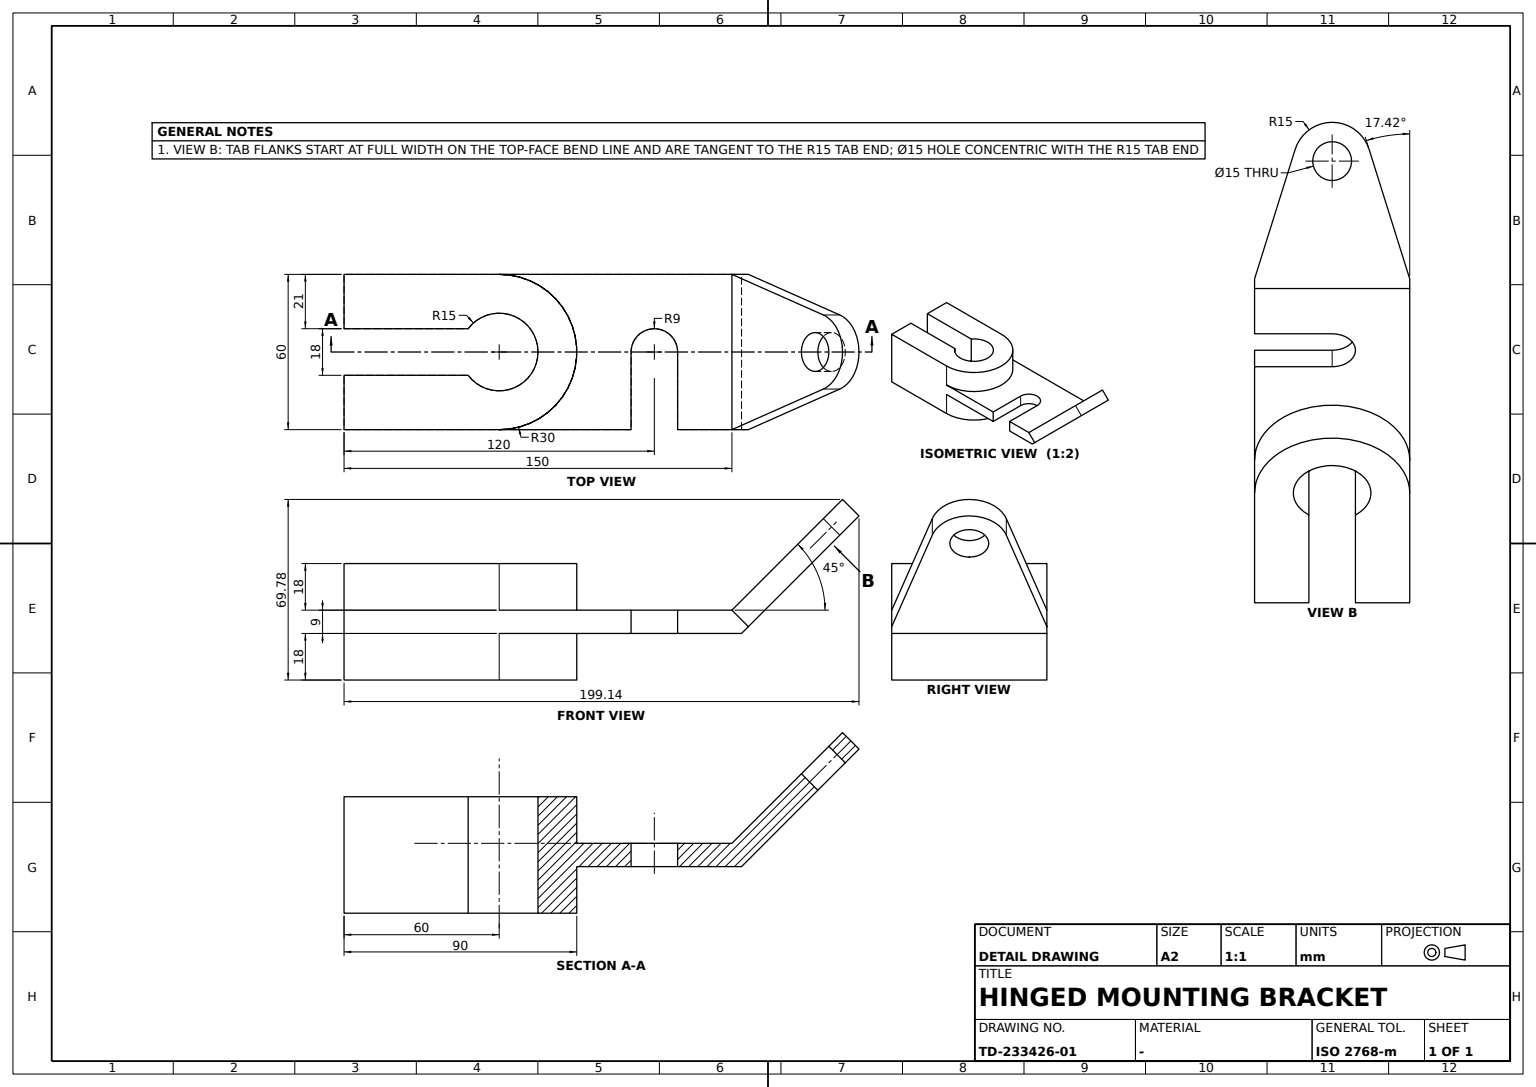
ISO-10303-21;
HEADER;
FILE_DESCRIPTION((''),'2;1');
FILE_NAME('','',(''),(''),'','','');
FILE_SCHEMA(('AUTOMOTIVE_DESIGN'));
ENDSEC;
DATA;
#1=APPLICATION_CONTEXT('');
#2=PRODUCT_CONTEXT('',#1,'mechanical');
#3=PRODUCT('','','',(#2));
#4=PRODUCT_DEFINITION_FORMATION('','',#3);
#5=PRODUCT_DEFINITION_CONTEXT('',#1,'design');
#6=PRODUCT_DEFINITION('','',#4,#5);
#7=PRODUCT_DEFINITION_SHAPE('','',#6);
#8=(LENGTH_UNIT()NAMED_UNIT(*)SI_UNIT(.MILLI.,.METRE.));
#9=(NAMED_UNIT(*)PLANE_ANGLE_UNIT()SI_UNIT($,.RADIAN.));
#10=(NAMED_UNIT(*)SI_UNIT($,.STERADIAN.)SOLID_ANGLE_UNIT());
#11=UNCERTAINTY_MEASURE_WITH_UNIT(LENGTH_MEASURE(0.005),#8,'distance_accuracy_value','');
#12=(GEOMETRIC_REPRESENTATION_CONTEXT(3)GLOBAL_UNCERTAINTY_ASSIGNED_CONTEXT((#11))GLOBAL_UNIT_ASSIGNED_CONTEXT((#8,#9,#10))REPRESENTATION_CONTEXT('',''));
#13=CARTESIAN_POINT('',(132.77996,0.,47.27996));
#14=VERTEX_POINT('',#13);
#15=CARTESIAN_POINT('',(125.349193,14.311818,39.849193));
#16=VERTEX_POINT('',#15);
#17=CARTESIAN_POINT('',(122.173359,0.,36.673359));
#18=DIRECTION('',(-0.707106781,0.,0.707106781));
#19=DIRECTION('',(0.707106781,0.,0.707106781));
#20=AXIS2_PLACEMENT_3D('',#17,#18,#19);
#21=CIRCLE('',#20,15.);
#22=EDGE_CURVE('',#14,#16,#21,.T.);
#23=ORIENTED_EDGE('',*,*,#22,.T.);
#24=CARTESIAN_POINT('',(90.,30.,4.5));
#25=VERTEX_POINT('',#24);
#26=DIRECTION('',(0.674665588,-0.299420588,0.674665588));
#27=VECTOR('',#26,1000.);
#28=LINE('',#24,#27);
#29=EDGE_CURVE('',#25,#16,#28,.T.);
#30=ORIENTED_EDGE('',*,*,#29,.F.);
#31=CARTESIAN_POINT('',(90.,-30.,4.5));
#32=VERTEX_POINT('',#31);
#33=DIRECTION('',(0.,1.,0.));
#34=VECTOR('',#33,1000.);
#35=LINE('',#31,#34);
#36=EDGE_CURVE('',#32,#25,#35,.T.);
#37=ORIENTED_EDGE('',*,*,#36,.F.);
#38=CARTESIAN_POINT('',(125.349193,-14.311818,39.849193));
#39=VERTEX_POINT('',#38);
#40=DIRECTION('',(-0.674665588,-0.299420588,-0.674665588));
#41=VECTOR('',#40,1000.);
#42=LINE('',#38,#41);
#43=EDGE_CURVE('',#39,#32,#42,.T.);
#44=ORIENTED_EDGE('',*,*,#43,.F.);
#45=EDGE_CURVE('',#39,#14,#21,.T.);
#46=ORIENTED_EDGE('',*,*,#45,.T.);
#47=EDGE_LOOP('',(#23,#30,#37,#44,#46));
#48=FACE_BOUND('',#47,.T.);
#49=CARTESIAN_POINT('',(127.476659,0.,41.976659));
#50=VERTEX_POINT('',#49);
#51=CARTESIAN_POINT('',(116.870058,0.,31.370058));
#52=VERTEX_POINT('',#51);
#53=AXIS2_PLACEMENT_3D('',#17,#18,#26);
#54=CIRCLE('',#53,7.5);
#55=EDGE_CURVE('',#50,#52,#54,.T.);
#56=ORIENTED_EDGE('',*,*,#55,.F.);
#57=EDGE_CURVE('',#52,#50,#54,.T.);
#58=ORIENTED_EDGE('',*,*,#57,.F.);
#59=EDGE_LOOP('',(#56,#58));
#60=FACE_BOUND('',#59,.T.);
#61=CARTESIAN_POINT('',(116.870058,-30.,31.370058));
#62=DIRECTION('',(0.707106781,0.,-0.707106781));
#63=DIRECTION('',(-0.707106781,0.,-0.707106781));
#64=AXIS2_PLACEMENT_3D('',#61,#62,#63);
#65=PLANE('',#64);
#66=ADVANCED_FACE('',(#48,#60),#65,.F.);
#67=ORIENTED_EDGE('',*,*,#55,.T.);
#68=CARTESIAN_POINT('',(123.234019,0.,25.006097));
#69=VERTEX_POINT('',#68);
#70=VECTOR('',#18,1000.);
#71=LINE('',#68,#70);
#72=EDGE_CURVE('',#69,#52,#71,.T.);
#73=ORIENTED_EDGE('',*,*,#72,.F.);
#74=CARTESIAN_POINT('',(133.84062,0.,35.612698));
#75=VERTEX_POINT('',#74);
#76=CARTESIAN_POINT('',(128.53732,0.,30.309398));
#77=AXIS2_PLACEMENT_3D('',#76,#18,#26);
#78=CIRCLE('',#77,7.5);
#79=EDGE_CURVE('',#75,#69,#78,.T.);
#80=ORIENTED_EDGE('',*,*,#79,.F.);
#81=LINE('',#74,#70);
#82=EDGE_CURVE('',#50,#75,#81,.F.);
#83=ORIENTED_EDGE('',*,*,#82,.F.);
#84=EDGE_LOOP('',(#67,#73,#80,#83));
#85=FACE_BOUND('',#84,.T.);
#86=AXIS2_PLACEMENT_3D('',#76,#18,#19);
#87=CYLINDRICAL_SURFACE('',#86,7.5);
#88=ADVANCED_FACE('',(#85),#87,.F.);
#89=CARTESIAN_POINT('',(51.,-30.,-4.5));
#90=VERTEX_POINT('',#89);
#91=CARTESIAN_POINT('',(51.,-30.,4.5));
#92=VERTEX_POINT('',#91);
#93=CARTESIAN_POINT('',(51.,-30.,-55.5));
#94=DIRECTION('',(0.,0.,1.));
#95=VECTOR('',#94,1000.);
#96=LINE('',#93,#95);
#97=EDGE_CURVE('',#90,#92,#96,.T.);
#98=ORIENTED_EDGE('',*,*,#97,.T.);
#99=CARTESIAN_POINT('',(0.,-30.,4.5));
#100=VERTEX_POINT('',#99);
#101=DIRECTION('',(-1.,0.,0.));
#102=VECTOR('',#101,1000.);
#103=LINE('',#31,#102);
#104=EDGE_CURVE('',#92,#100,#103,.T.);
#105=ORIENTED_EDGE('',*,*,#104,.T.);
#106=CARTESIAN_POINT('',(0.,-30.,22.5));
#107=VERTEX_POINT('',#106);
#108=DIRECTION('',(0.,0.,-1.));
#109=VECTOR('',#108,1000.);
#110=LINE('',#106,#109);
#111=EDGE_CURVE('',#107,#100,#110,.T.);
#112=ORIENTED_EDGE('',*,*,#111,.F.);
#113=CARTESIAN_POINT('',(-60.,-30.,22.5));
#114=VERTEX_POINT('',#113);
#115=DIRECTION('',(1.,0.,0.));
#116=VECTOR('',#115,1000.);
#117=LINE('',#113,#116);
#118=EDGE_CURVE('',#114,#107,#117,.T.);
#119=ORIENTED_EDGE('',*,*,#118,.F.);
#120=CARTESIAN_POINT('',(-60.,-30.,-22.5));
#121=VERTEX_POINT('',#120);
#122=LINE('',#113,#109);
#123=EDGE_CURVE('',#114,#121,#122,.T.);
#124=ORIENTED_EDGE('',*,*,#123,.T.);
#125=CARTESIAN_POINT('',(0.,-30.,-22.5));
#126=VERTEX_POINT('',#125);
#127=LINE('',#120,#116);
#128=EDGE_CURVE('',#121,#126,#127,.T.);
#129=ORIENTED_EDGE('',*,*,#128,.T.);
#130=CARTESIAN_POINT('',(0.,-30.,-4.5));
#131=VERTEX_POINT('',#130);
#132=EDGE_CURVE('',#131,#126,#110,.T.);
#133=ORIENTED_EDGE('',*,*,#132,.F.);
#134=LINE('',#130,#116);
#135=EDGE_CURVE('',#131,#90,#134,.T.);
#136=ORIENTED_EDGE('',*,*,#135,.T.);
#137=EDGE_LOOP('',(#98,#105,#112,#119,#124,#129,#133,#136));
#138=FACE_BOUND('',#137,.T.);
#139=AXIS2_PLACEMENT_3D('',#113,#33,#94);
#140=PLANE('',#139);
#141=ADVANCED_FACE('',(#138),#140,.F.);
#142=CARTESIAN_POINT('',(69.,0.,4.5));
#143=VERTEX_POINT('',#142);
#144=CARTESIAN_POINT('',(51.,0.,4.5));
#145=VERTEX_POINT('',#144);
#146=CARTESIAN_POINT('',(60.,0.,4.5));
#147=AXIS2_PLACEMENT_3D('',#146,#94,#115);
#148=CIRCLE('',#147,9.);
#149=EDGE_CURVE('',#143,#145,#148,.T.);
#150=ORIENTED_EDGE('',*,*,#149,.F.);
#151=CARTESIAN_POINT('',(69.,-30.,4.5));
#152=VERTEX_POINT('',#151);
#153=LINE('',#151,#34);
#154=EDGE_CURVE('',#152,#143,#153,.T.);
#155=ORIENTED_EDGE('',*,*,#154,.F.);
#156=EDGE_CURVE('',#32,#152,#103,.T.);
#157=ORIENTED_EDGE('',*,*,#156,.F.);
#158=ORIENTED_EDGE('',*,*,#36,.T.);
#159=CARTESIAN_POINT('',(0.,30.,4.5));
#160=VERTEX_POINT('',#159);
#161=LINE('',#24,#102);
#162=EDGE_CURVE('',#25,#160,#161,.T.);
#163=ORIENTED_EDGE('',*,*,#162,.T.);
#164=CARTESIAN_POINT('',(0.,0.,4.5));
#165=AXIS2_PLACEMENT_3D('',#164,#108,#101);
#166=CIRCLE('',#165,30.);
#167=EDGE_CURVE('',#160,#100,#166,.T.);
#168=ORIENTED_EDGE('',*,*,#167,.T.);
#169=ORIENTED_EDGE('',*,*,#104,.F.);
#170=DIRECTION('',(0.,-1.,0.));
#171=VECTOR('',#170,1000.);
#172=LINE('',#144,#171);
#173=EDGE_CURVE('',#145,#92,#172,.T.);
#174=ORIENTED_EDGE('',*,*,#173,.F.);
#175=EDGE_LOOP('',(#150,#155,#157,#158,#163,#168,#169,#174));
#176=FACE_BOUND('',#175,.T.);
#177=AXIS2_PLACEMENT_3D('',#31,#108,#101);
#178=PLANE('',#177);
#179=ADVANCED_FACE('',(#176),#178,.F.);
#180=ORIENTED_EDGE('',*,*,#79,.T.);
#181=EDGE_CURVE('',#69,#75,#78,.T.);
#182=ORIENTED_EDGE('',*,*,#181,.T.);
#183=EDGE_LOOP('',(#180,#182));
#184=FACE_BOUND('',#183,.T.);
#185=CARTESIAN_POINT('',(93.727922,-30.,-4.5));
#186=VERTEX_POINT('',#185);
#187=CARTESIAN_POINT('',(96.363961,-30.,-1.863961));
#188=VERTEX_POINT('',#187);
#189=VECTOR('',#19,1000.);
#190=LINE('',#185,#189);
#191=EDGE_CURVE('',#186,#188,#190,.T.);
#192=ORIENTED_EDGE('',*,*,#191,.F.);
#193=CARTESIAN_POINT('',(93.727922,30.,-4.5));
#194=VERTEX_POINT('',#193);
#195=LINE('',#185,#34);
#196=EDGE_CURVE('',#186,#194,#195,.T.);
#197=ORIENTED_EDGE('',*,*,#196,.T.);
#198=CARTESIAN_POINT('',(96.363961,30.,-1.863961));
#199=VERTEX_POINT('',#198);
#200=LINE('',#193,#189);
#201=EDGE_CURVE('',#194,#199,#200,.T.);
#202=ORIENTED_EDGE('',*,*,#201,.T.);
#203=CARTESIAN_POINT('',(131.713154,14.311818,33.485232));
#204=VERTEX_POINT('',#203);
#205=LINE('',#198,#27);
#206=EDGE_CURVE('',#199,#204,#205,.T.);
#207=ORIENTED_EDGE('',*,*,#206,.T.);
#208=CARTESIAN_POINT('',(139.143921,0.,40.915999));
#209=VERTEX_POINT('',#208);
#210=CIRCLE('',#86,15.);
#211=EDGE_CURVE('',#209,#204,#210,.T.);
#212=ORIENTED_EDGE('',*,*,#211,.F.);
#213=CARTESIAN_POINT('',(131.713154,-14.311818,33.485232));
#214=VERTEX_POINT('',#213);
#215=EDGE_CURVE('',#214,#209,#210,.T.);
#216=ORIENTED_EDGE('',*,*,#215,.F.);
#217=LINE('',#213,#41);
#218=EDGE_CURVE('',#214,#188,#217,.T.);
#219=ORIENTED_EDGE('',*,*,#218,.T.);
#220=EDGE_LOOP('',(#192,#197,#202,#207,#212,#216,#219));
#221=FACE_BOUND('',#220,.T.);
#222=AXIS2_PLACEMENT_3D('',#185,#18,#19);
#223=PLANE('',#222);
#224=ADVANCED_FACE('',(#184,#221),#223,.F.);
#225=CARTESIAN_POINT('',(-12.,9.,-22.5));
#226=VERTEX_POINT('',#225);
#227=CARTESIAN_POINT('',(-60.,9.,-22.5));
#228=VERTEX_POINT('',#227);
#229=CARTESIAN_POINT('',(8.,9.,-22.5));
#230=LINE('',#229,#102);
#231=EDGE_CURVE('',#226,#228,#230,.T.);
#232=ORIENTED_EDGE('',*,*,#231,.T.);
#233=CARTESIAN_POINT('',(-60.,30.,-22.5));
#234=VERTEX_POINT('',#233);
#235=LINE('',#233,#171);
#236=EDGE_CURVE('',#234,#228,#235,.T.);
#237=ORIENTED_EDGE('',*,*,#236,.F.);
#238=CARTESIAN_POINT('',(0.,30.,-22.5));
#239=VERTEX_POINT('',#238);
#240=LINE('',#238,#102);
#241=EDGE_CURVE('',#239,#234,#240,.T.);
#242=ORIENTED_EDGE('',*,*,#241,.F.);
#243=CARTESIAN_POINT('',(0.,0.,-22.5));
#244=AXIS2_PLACEMENT_3D('',#243,#94,#115);
#245=CIRCLE('',#244,30.);
#246=EDGE_CURVE('',#126,#239,#245,.T.);
#247=ORIENTED_EDGE('',*,*,#246,.F.);
#248=ORIENTED_EDGE('',*,*,#128,.F.);
#249=CARTESIAN_POINT('',(-60.,-9.,-22.5));
#250=VERTEX_POINT('',#249);
#251=EDGE_CURVE('',#250,#121,#235,.T.);
#252=ORIENTED_EDGE('',*,*,#251,.F.);
#253=CARTESIAN_POINT('',(-12.,-9.,-22.5));
#254=VERTEX_POINT('',#253);
#255=LINE('',#249,#116);
#256=EDGE_CURVE('',#250,#254,#255,.T.);
#257=ORIENTED_EDGE('',*,*,#256,.T.);
#258=CARTESIAN_POINT('',(15.,0.,-22.5));
#259=VERTEX_POINT('',#258);
#260=AXIS2_PLACEMENT_3D('',#243,#94,#33);
#261=CIRCLE('',#260,15.);
#262=EDGE_CURVE('',#254,#259,#261,.T.);
#263=ORIENTED_EDGE('',*,*,#262,.T.);
#264=EDGE_CURVE('',#259,#226,#261,.T.);
#265=ORIENTED_EDGE('',*,*,#264,.T.);
#266=EDGE_LOOP('',(#232,#237,#242,#247,#248,#252,#257,#263,#265));
#267=FACE_BOUND('',#266,.T.);
#268=PLANE('',#244);
#269=ADVANCED_FACE('',(#267),#268,.F.);
#270=CARTESIAN_POINT('',(0.,30.,22.5));
#271=VERTEX_POINT('',#270);
#272=LINE('',#270,#109);
#273=EDGE_CURVE('',#271,#160,#272,.T.);
#274=ORIENTED_EDGE('',*,*,#273,.F.);
#275=CARTESIAN_POINT('',(0.,0.,22.5));
#276=AXIS2_PLACEMENT_3D('',#275,#94,#115);
#277=CIRCLE('',#276,30.);
#278=EDGE_CURVE('',#107,#271,#277,.T.);
#279=ORIENTED_EDGE('',*,*,#278,.F.);
#280=ORIENTED_EDGE('',*,*,#111,.T.);
#281=ORIENTED_EDGE('',*,*,#167,.F.);
#282=EDGE_LOOP('',(#274,#279,#280,#281));
#283=FACE_BOUND('',#282,.T.);
#284=AXIS2_PLACEMENT_3D('',#275,#108,#101);
#285=CYLINDRICAL_SURFACE('',#284,30.);
#286=ADVANCED_FACE('',(#283),#285,.T.);
#287=ORIENTED_EDGE('',*,*,#29,.T.);
#288=LINE('',#203,#70);
#289=EDGE_CURVE('',#204,#16,#288,.T.);
#290=ORIENTED_EDGE('',*,*,#289,.F.);
#291=ORIENTED_EDGE('',*,*,#206,.F.);
#292=LINE('',#198,#70);
#293=EDGE_CURVE('',#199,#25,#292,.T.);
#294=ORIENTED_EDGE('',*,*,#293,.T.);
#295=EDGE_LOOP('',(#287,#290,#291,#294));
#296=FACE_BOUND('',#295,.T.);
#297=DIRECTION('',(-0.211722328,-0.954121225,-0.211722328));
#298=DIRECTION('',(0.976253017,-0.216633438,0.));
#299=AXIS2_PLACEMENT_3D('',#198,#297,#298);
#300=PLANE('',#299);
#301=ADVANCED_FACE('',(#296),#300,.F.);
#302=CARTESIAN_POINT('',(0.,30.,-4.5));
#303=VERTEX_POINT('',#302);
#304=EDGE_CURVE('',#303,#239,#272,.T.);
#305=ORIENTED_EDGE('',*,*,#304,.T.);
#306=ORIENTED_EDGE('',*,*,#241,.T.);
#307=CARTESIAN_POINT('',(-60.,30.,22.5));
#308=VERTEX_POINT('',#307);
#309=LINE('',#307,#109);
#310=EDGE_CURVE('',#308,#234,#309,.T.);
#311=ORIENTED_EDGE('',*,*,#310,.F.);
#312=LINE('',#270,#102);
#313=EDGE_CURVE('',#271,#308,#312,.T.);
#314=ORIENTED_EDGE('',*,*,#313,.F.);
#315=ORIENTED_EDGE('',*,*,#273,.T.);
#316=ORIENTED_EDGE('',*,*,#162,.F.);
#317=ORIENTED_EDGE('',*,*,#293,.F.);
#318=ORIENTED_EDGE('',*,*,#201,.F.);
#319=LINE('',#302,#116);
#320=EDGE_CURVE('',#303,#194,#319,.T.);
#321=ORIENTED_EDGE('',*,*,#320,.F.);
#322=EDGE_LOOP('',(#305,#306,#311,#314,#315,#316,#317,#318,#321));
#323=FACE_BOUND('',#322,.T.);
#324=AXIS2_PLACEMENT_3D('',#270,#170,#108);
#325=PLANE('',#324);
#326=ADVANCED_FACE('',(#323),#325,.F.);
#327=ORIENTED_EDGE('',*,*,#231,.F.);
#328=CARTESIAN_POINT('',(-12.,9.,22.5));
#329=VERTEX_POINT('',#328);
#330=LINE('',#225,#109);
#331=EDGE_CURVE('',#329,#226,#330,.T.);
#332=ORIENTED_EDGE('',*,*,#331,.F.);
#333=CARTESIAN_POINT('',(-60.,9.,22.5));
#334=VERTEX_POINT('',#333);
#335=CARTESIAN_POINT('',(8.,9.,22.5));
#336=LINE('',#335,#102);
#337=EDGE_CURVE('',#329,#334,#336,.T.);
#338=ORIENTED_EDGE('',*,*,#337,.T.);
#339=LINE('',#227,#95);
#340=EDGE_CURVE('',#228,#334,#339,.T.);
#341=ORIENTED_EDGE('',*,*,#340,.F.);
#342=EDGE_LOOP('',(#327,#332,#338,#341));
#343=FACE_BOUND('',#342,.T.);
#344=AXIS2_PLACEMENT_3D('',#229,#33,#101);
#345=PLANE('',#344);
#346=ADVANCED_FACE('',(#343),#345,.F.);
#347=ORIENTED_EDGE('',*,*,#246,.T.);
#348=ORIENTED_EDGE('',*,*,#304,.F.);
#349=CARTESIAN_POINT('',(0.,0.,-4.5));
#350=AXIS2_PLACEMENT_3D('',#349,#94,#115);
#351=CIRCLE('',#350,30.);
#352=EDGE_CURVE('',#131,#303,#351,.T.);
#353=ORIENTED_EDGE('',*,*,#352,.F.);
#354=ORIENTED_EDGE('',*,*,#132,.T.);
#355=EDGE_LOOP('',(#347,#348,#353,#354));
#356=FACE_BOUND('',#355,.T.);
#357=ADVANCED_FACE('',(#356),#285,.T.);
#358=ORIENTED_EDGE('',*,*,#57,.T.);
#359=ORIENTED_EDGE('',*,*,#82,.T.);
#360=ORIENTED_EDGE('',*,*,#181,.F.);
#361=ORIENTED_EDGE('',*,*,#72,.T.);
#362=EDGE_LOOP('',(#358,#359,#360,#361));
#363=FACE_BOUND('',#362,.T.);
#364=ADVANCED_FACE('',(#363),#87,.F.);
#365=CARTESIAN_POINT('',(-12.,-9.,22.5));
#366=VERTEX_POINT('',#365);
#367=LINE('',#253,#95);
#368=EDGE_CURVE('',#254,#366,#367,.T.);
#369=ORIENTED_EDGE('',*,*,#368,.F.);
#370=ORIENTED_EDGE('',*,*,#256,.F.);
#371=CARTESIAN_POINT('',(-60.,-9.,22.5));
#372=VERTEX_POINT('',#371);
#373=LINE('',#249,#95);
#374=EDGE_CURVE('',#250,#372,#373,.T.);
#375=ORIENTED_EDGE('',*,*,#374,.T.);
#376=LINE('',#371,#116);
#377=EDGE_CURVE('',#372,#366,#376,.T.);
#378=ORIENTED_EDGE('',*,*,#377,.T.);
#379=EDGE_LOOP('',(#369,#370,#375,#378));
#380=FACE_BOUND('',#379,.T.);
#381=AXIS2_PLACEMENT_3D('',#249,#170,#115);
#382=PLANE('',#381);
#383=ADVANCED_FACE('',(#380),#382,.F.);
#384=CARTESIAN_POINT('',(51.,0.,-4.5));
#385=VERTEX_POINT('',#384);
#386=CARTESIAN_POINT('',(51.,0.,-55.5));
#387=LINE('',#386,#109);
#388=EDGE_CURVE('',#145,#385,#387,.T.);
#389=ORIENTED_EDGE('',*,*,#388,.F.);
#390=ORIENTED_EDGE('',*,*,#173,.T.);
#391=ORIENTED_EDGE('',*,*,#97,.F.);
#392=LINE('',#89,#171);
#393=EDGE_CURVE('',#385,#90,#392,.T.);
#394=ORIENTED_EDGE('',*,*,#393,.F.);
#395=EDGE_LOOP('',(#389,#390,#391,#394));
#396=FACE_BOUND('',#395,.T.);
#397=AXIS2_PLACEMENT_3D('',#386,#101,#170);
#398=PLANE('',#397);
#399=ADVANCED_FACE('',(#396),#398,.F.);
#400=ORIENTED_EDGE('',*,*,#236,.T.);
#401=ORIENTED_EDGE('',*,*,#340,.T.);
#402=LINE('',#307,#171);
#403=EDGE_CURVE('',#308,#334,#402,.T.);
#404=ORIENTED_EDGE('',*,*,#403,.F.);
#405=ORIENTED_EDGE('',*,*,#310,.T.);
#406=EDGE_LOOP('',(#400,#401,#404,#405));
#407=FACE_BOUND('',#406,.T.);
#408=AXIS2_PLACEMENT_3D('',#307,#115,#108);
#409=PLANE('',#408);
#410=ADVANCED_FACE('',(#407),#409,.F.);
#411=ORIENTED_EDGE('',*,*,#374,.F.);
#412=ORIENTED_EDGE('',*,*,#251,.T.);
#413=ORIENTED_EDGE('',*,*,#123,.F.);
#414=EDGE_CURVE('',#372,#114,#402,.T.);
#415=ORIENTED_EDGE('',*,*,#414,.F.);
#416=EDGE_LOOP('',(#411,#412,#413,#415));
#417=FACE_BOUND('',#416,.T.);
#418=ADVANCED_FACE('',(#417),#409,.F.);
#419=CARTESIAN_POINT('',(15.,0.,22.5));
#420=VERTEX_POINT('',#419);
#421=AXIS2_PLACEMENT_3D('',#275,#94,#33);
#422=CIRCLE('',#421,15.);
#423=EDGE_CURVE('',#366,#420,#422,.T.);
#424=ORIENTED_EDGE('',*,*,#423,.T.);
#425=LINE('',#258,#95);
#426=EDGE_CURVE('',#259,#420,#425,.T.);
#427=ORIENTED_EDGE('',*,*,#426,.F.);
#428=ORIENTED_EDGE('',*,*,#262,.F.);
#429=ORIENTED_EDGE('',*,*,#368,.T.);
#430=EDGE_LOOP('',(#424,#427,#428,#429));
#431=FACE_BOUND('',#430,.T.);
#432=CYLINDRICAL_SURFACE('',#244,15.);
#433=ADVANCED_FACE('',(#431),#432,.F.);
#434=ORIENTED_EDGE('',*,*,#22,.F.);
#435=LINE('',#208,#70);
#436=EDGE_CURVE('',#209,#14,#435,.T.);
#437=ORIENTED_EDGE('',*,*,#436,.F.);
#438=ORIENTED_EDGE('',*,*,#211,.T.);
#439=ORIENTED_EDGE('',*,*,#289,.T.);
#440=EDGE_LOOP('',(#434,#437,#438,#439));
#441=FACE_BOUND('',#440,.T.);
#442=CYLINDRICAL_SURFACE('',#86,15.);
#443=ADVANCED_FACE('',(#441),#442,.T.);
#444=EDGE_CURVE('',#420,#329,#422,.T.);
#445=ORIENTED_EDGE('',*,*,#444,.T.);
#446=ORIENTED_EDGE('',*,*,#331,.T.);
#447=ORIENTED_EDGE('',*,*,#264,.F.);
#448=ORIENTED_EDGE('',*,*,#426,.T.);
#449=EDGE_LOOP('',(#445,#446,#447,#448));
#450=FACE_BOUND('',#449,.T.);
#451=ADVANCED_FACE('',(#450),#432,.F.);
#452=ORIENTED_EDGE('',*,*,#45,.F.);
#453=LINE('',#213,#70);
#454=EDGE_CURVE('',#214,#39,#453,.T.);
#455=ORIENTED_EDGE('',*,*,#454,.F.);
#456=ORIENTED_EDGE('',*,*,#215,.T.);
#457=ORIENTED_EDGE('',*,*,#436,.T.);
#458=EDGE_LOOP('',(#452,#455,#456,#457));
#459=FACE_BOUND('',#458,.T.);
#460=ADVANCED_FACE('',(#459),#442,.T.);
#461=ORIENTED_EDGE('',*,*,#414,.T.);
#462=ORIENTED_EDGE('',*,*,#118,.T.);
#463=ORIENTED_EDGE('',*,*,#278,.T.);
#464=ORIENTED_EDGE('',*,*,#313,.T.);
#465=ORIENTED_EDGE('',*,*,#403,.T.);
#466=ORIENTED_EDGE('',*,*,#337,.F.);
#467=ORIENTED_EDGE('',*,*,#444,.F.);
#468=ORIENTED_EDGE('',*,*,#423,.F.);
#469=ORIENTED_EDGE('',*,*,#377,.F.);
#470=EDGE_LOOP('',(#461,#462,#463,#464,#465,#466,#467,#468,#469));
#471=FACE_BOUND('',#470,.T.);
#472=PLANE('',#276);
#473=ADVANCED_FACE('',(#471),#472,.T.);
#474=ORIENTED_EDGE('',*,*,#218,.F.);
#475=ORIENTED_EDGE('',*,*,#454,.T.);
#476=ORIENTED_EDGE('',*,*,#43,.T.);
#477=LINE('',#187,#70);
#478=EDGE_CURVE('',#188,#32,#477,.T.);
#479=ORIENTED_EDGE('',*,*,#478,.F.);
#480=EDGE_LOOP('',(#474,#475,#476,#479));
#481=FACE_BOUND('',#480,.T.);
#482=DIRECTION('',(-0.211722328,0.954121225,-0.211722328));
#483=DIRECTION('',(-0.976253017,-0.216633438,0.));
#484=AXIS2_PLACEMENT_3D('',#213,#482,#483);
#485=PLANE('',#484);
#486=ADVANCED_FACE('',(#481),#485,.F.);
#487=CARTESIAN_POINT('',(69.,-30.,-4.5));
#488=VERTEX_POINT('',#487);
#489=CARTESIAN_POINT('',(69.,0.,-4.5));
#490=VERTEX_POINT('',#489);
#491=LINE('',#487,#34);
#492=EDGE_CURVE('',#488,#490,#491,.T.);
#493=ORIENTED_EDGE('',*,*,#492,.F.);
#494=CARTESIAN_POINT('',(69.,-30.,-55.5));
#495=LINE('',#494,#95);
#496=EDGE_CURVE('',#488,#152,#495,.T.);
#497=ORIENTED_EDGE('',*,*,#496,.T.);
#498=ORIENTED_EDGE('',*,*,#154,.T.);
#499=CARTESIAN_POINT('',(69.,0.,-55.5));
#500=LINE('',#499,#109);
#501=EDGE_CURVE('',#143,#490,#500,.T.);
#502=ORIENTED_EDGE('',*,*,#501,.T.);
#503=EDGE_LOOP('',(#493,#497,#498,#502));
#504=FACE_BOUND('',#503,.T.);
#505=AXIS2_PLACEMENT_3D('',#494,#115,#33);
#506=PLANE('',#505);
#507=ADVANCED_FACE('',(#504),#506,.F.);
#508=ORIENTED_EDGE('',*,*,#135,.F.);
#509=ORIENTED_EDGE('',*,*,#352,.T.);
#510=ORIENTED_EDGE('',*,*,#320,.T.);
#511=ORIENTED_EDGE('',*,*,#196,.F.);
#512=EDGE_CURVE('',#488,#186,#134,.T.);
#513=ORIENTED_EDGE('',*,*,#512,.F.);
#514=ORIENTED_EDGE('',*,*,#492,.T.);
#515=CARTESIAN_POINT('',(60.,0.,-4.5));
#516=AXIS2_PLACEMENT_3D('',#515,#94,#115);
#517=CIRCLE('',#516,9.);
#518=EDGE_CURVE('',#490,#385,#517,.T.);
#519=ORIENTED_EDGE('',*,*,#518,.T.);
#520=ORIENTED_EDGE('',*,*,#393,.T.);
#521=EDGE_LOOP('',(#508,#509,#510,#511,#513,#514,#519,#520));
#522=FACE_BOUND('',#521,.T.);
#523=AXIS2_PLACEMENT_3D('',#130,#94,#115);
#524=PLANE('',#523);
#525=ADVANCED_FACE('',(#522),#524,.F.);
#526=ORIENTED_EDGE('',*,*,#156,.T.);
#527=ORIENTED_EDGE('',*,*,#496,.F.);
#528=ORIENTED_EDGE('',*,*,#512,.T.);
#529=ORIENTED_EDGE('',*,*,#191,.T.);
#530=ORIENTED_EDGE('',*,*,#478,.T.);
#531=EDGE_LOOP('',(#526,#527,#528,#529,#530));
#532=FACE_BOUND('',#531,.T.);
#533=ADVANCED_FACE('',(#532),#140,.F.);
#534=ORIENTED_EDGE('',*,*,#388,.T.);
#535=ORIENTED_EDGE('',*,*,#518,.F.);
#536=ORIENTED_EDGE('',*,*,#501,.F.);
#537=ORIENTED_EDGE('',*,*,#149,.T.);
#538=EDGE_LOOP('',(#534,#535,#536,#537));
#539=FACE_BOUND('',#538,.T.);
#540=CARTESIAN_POINT('',(60.,0.,-55.5));
#541=AXIS2_PLACEMENT_3D('',#540,#94,#115);
#542=CYLINDRICAL_SURFACE('',#541,9.);
#543=ADVANCED_FACE('',(#539),#542,.F.);
#544=CLOSED_SHELL('',(#66,#88,#141,#179,#224,#269,#286,#301,#326,#346,#357,#364,#383,#399,#410,#418,#433,#443,#451,#460,#473,#486,#507,#525,#533,#543));
#545=MANIFOLD_SOLID_BREP('',#544);
#546=ADVANCED_BREP_SHAPE_REPRESENTATION('',(#545),#12);
#547=SHAPE_DEFINITION_REPRESENTATION(#7,#546);
ENDSEC;
END-ISO-10303-21;
